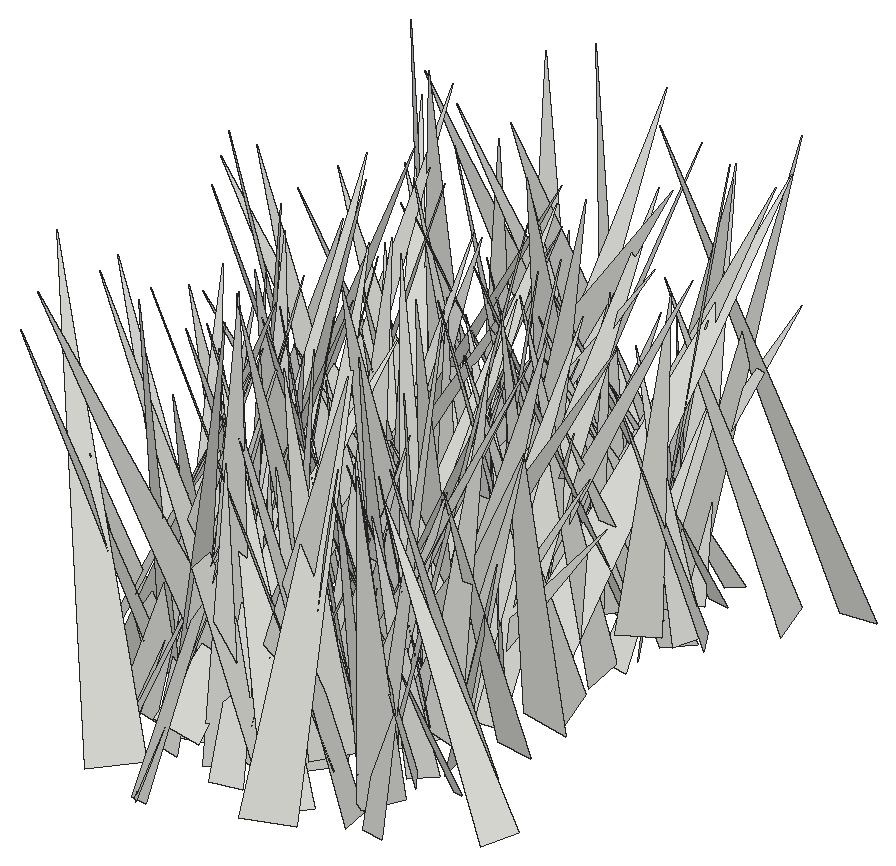
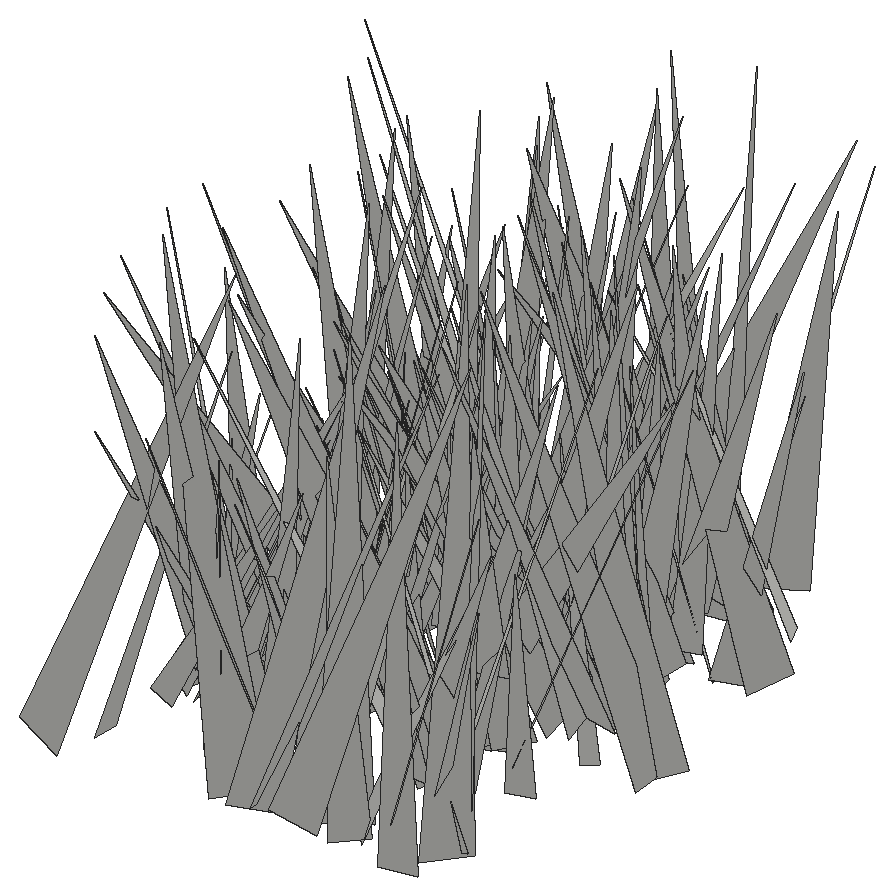
# SketchUp Ruby script. Lengths in inches.
U = 1.inch
M = Sketchup.active_model
def pt(a) = Geom::Point3d.new(a.map { |v| v * U })
def face(e, loops, mat)
  f = e.add_face(loops[0].map { |a| pt(a) })
  loops[1..].each { |l| e.add_face(l.map { |a| pt(a) }).erase! }
  f.material = f.back_material = mat if mat
  f
end
# faces: each face lists its corners as indices into pts; further lists are holes
def faces(e, pts, list, mat = nil) = list.each { |f| face(e, (f[0].is_a?(Array) ? f : [f]).map { |l| l.map { |i| pts[i] } }, mat) }
# xy, xz, yz: faces in a plane at the given z, y or x. An outline is a flat list of corners, or four numbers for a rectangle; further outlines are holes
def ring(l) = l.size == 4 ? [[l[0], l[1]], [l[2], l[1]], [l[2], l[3]], [l[0], l[3]]] : l.each_slice(2).to_a
def flat(e, list, mat, &to3) = list.each { |f| face(e, (f[0].is_a?(Array) ? f : [f]).map { |l| ring(l).map { |u, v| to3.(u, v) } }, mat) }
def xy(e, z, list, mat = nil) = flat(e, list, mat) { |x, y| [x, y, z] }
def xz(e, y, list, mat = nil) = flat(e, list, mat) { |x, z| [x, y, z] }
def yz(e, x, list, mat = nil) = flat(e, list, mat) { |y, z| [x, y, z] }
def lines(e, pts, list) = list.each { |a, b| e.add_line(pt(pts[a]), pt(pts[b])) }
# prism: a flat outline (further loops are holes) pulled along v
def prism(e, loops, v, mat = nil)
  f = face(e, loops, mat); d = Geom::Vector3d.new(v.map { |x| x * U })
  f.pushpull(f.normal.samedirection?(d) ? d.length : -d.length)
end
def box(e, o, s, mat = nil) = prism(e, [[o, [o[0] + s[0], o[1], o[2]], [o[0] + s[0], o[1] + s[1], o[2]], [o[0], o[1] + s[1], o[2]]]], [0, 0, s[2]], mat)
def at(x, y, z, deg = 0) = Geom::Transformation.translation(pt([x, y, z])) * Geom::Transformation.rotation(ORIGIN, Z_AXIS, deg.degrees)
def axes(o, x, y, z) = Geom::Transformation.new([*x, 0, *y, 0, *z, 0, *pt(o).to_a, 1])
def part(name) = M.definitions.add(name)
# library, detail: a bought-in or finely detailed component or shape, given as its bounding box
def library(name, o, s) = part(name).tap { |d| box(d.entities, o, s) }
def detail(e, o, s) = box(e.add_group.entities, o, s)
def put(e, d, t, mat = nil) = e.add_instance(d, t).tap { |i| i.material = mat if mat }
def group(e, t, mat = nil) = e.add_group.tap { |g| g.transformation = t; g.material = mat if mat }.entities
root = M.entities
c1 = part("fur_instance\#9")
p = [[0.8125,0,1.79],[0.67,-0.02,1.48],[0,-0.11,0],[0,0.11,0]]
faces(c1.entities,p,[[0,1,2,3]])
put(root,c1,axes([88.71,113.59,-28.22],[3.36953,-3.09183,0.80409],[-2.80421,-3.42236,-1.4084],[-1.53048,-0.53643,4.35081]))
put(root,c1,axes([89.1875,126.13,-28.22],[-3.67755,-0.2078,1.11626],[-0.0694,3.8179,0.48208],[1.13331,-0.4405,3.65173]))
put(root,c1,axes([89.17,122.14,-28.22],[-1.55614,3.71904,0.91385],[3.82438,1.56093,0.15988],[0.20123,-0.90564,4.0283]))
put(root,c1,axes([90.7,112.91,-27.1],[-5.38349,2.8617,0.60302],[2.91403,5.35589,0.59819],[0.24775,-0.81245,6.06741]))
put(root,c1,axes([90.85,108.57,-28.22],[-5.24663,5.623,0.95369],[5.70188,5.20042,0.70642],[0.12741,-1.17997,7.65808]))
put(root,c1,axes([88.99,124.78,-27.1],[-4.49865,-5.44108,2.87885],[-5.83326,4.90701,0.15896],[1.96626,2.10876,7.05818]))
put(root,c1,axes([90.92,124.77,-27.1],[-2.13288,4.47426,0.69403],[4.36785,1.83113,1.61826],[-1.19274,-1.2953,4.68502]))
put(root,c1,axes([86.76,118.93,-28.22],[5.41416,-4.66063,0.97473],[-4.76032,-5.26587,1.26282],[0.1044,1.59183,7.03135]))
put(root,c1,axes([89.56,112.2,-27.1],[-5.06426,-4.56399,0.84014],[-4.29824,5.08189,1.69768],[1.74956,-0.72593,6.60262]))
put(root,c1,axes([89.875,124.81,-28.22],[-5.39374,-4.42373,0.73063],[-4.15874,5.36317,1.77113],[1.67573,-0.92879,6.74722]))
put(root,c1,axes([89.88,126.89,-27.1],[-3.92886,-2.51502,0.86647],[-2.44083,4.02285,0.60923],[1.05758,-0.05874,4.62495]))
put(root,c1,axes([86.84,119.02,-28.22],[7.79072,-0.23447,0.87822],[-0.35324,-7.76347,1.06082],[-0.83754,1.09323,7.72172]))
put(root,c1,axes([92.92,120.51,-28.22],[-4.16636,5.9481,1.52453],[5.74666,3.12806,3.50054],[-2.16332,-3.14611,6.36276]))
put(root,c1,axes([91.7,117.82,-27.1],[-6.3033,-3.29184,1.05702],[-3.45211,6.11366,-1.54635],[0.19083,1.86335,6.94094]))
put(root,c1,axes([90.43,120.77,-28.22],[-5.31145,-3.30369,0.30508],[-3.10318,5.15062,1.7494],[1.17379,-1.33255,6.00546]))
put(root,c1,axes([88.53,117.63,-28.22],[6.37942,2.61315,2.43113],[3.05762,-6.56979,-0.96169],[-1.84118,-1.85616,6.82648]))
put(root,c1,axes([91.35,126.52,-28.22],[-3.75562,-3.58045,0.3486],[-3.58145,3.67402,-0.84892],[-0.33818,0.85312,5.11895]))
put(root,c1,axes([88.83,119.2,-27.1],[1.55056,7.17303,0.47228],[7.18686,-1.53634,-0.26142],[0.15632,-0.51668,7.33405]))
put(root,c1,axes([89.91,115.51,-28.22],[2.88835,4.68484,1.93004],[4.79823,-3.24275,0.69058],[-1.62782,-1.24585,5.46016]))
put(root,c1,axes([88.52,126.21,-28.22],[7.55718,-3.05255,1.8054],[-2.7949,-7.74218,-1.39129],[-2.18313,-0.65505,8.03077]))
put(root,c1,axes([90.47,115.76,-28.22],[3.4747,-4.84053,2.29693],[-4.84614,-4.00697,-1.11322],[-2.28507,1.13736,5.85363]))
put(root,c1,axes([88.5,125.73,-28.22],[-0.2038,-3.57727,1.86557],[-3.68837,0.92217,1.36537],[1.63497,1.63446,3.31273]))
put(root,c1,axes([91.42,120.62,-28.22],[-3.35316,6.39569,0.22234],[6.39729,3.34326,0.30873],[-0.17041,-0.34016,7.2148]))
put(root,c1,axes([90.11,116.29,-28.22],[-2.28357,5.70644,2.33564],[6.0895,2.47813,-0.10083],[0.96778,-2.12809,6.14557]))
put(root,c1,axes([89.13,127.62,-28.22],[0.11264,-6.37998,1.60761],[-6.5012,0.13924,1.0081],[1.01142,1.60553,6.30084]))
put(root,c1,axes([91.64,122.14,-27.1],[-5.50696,2.25656,1.40845],[2.52369,5.45565,1.12666],[0.84072,-1.59571,5.84374]))
put(root,c1,axes([87.69,111.89,-27.1],[5.0651,3.0377,0.15182],[3.00547,-4.95362,-1.15532],[0.46672,-1.0677,5.79207]))
put(root,c1,axes([90.78,122.63,-28.22],[-1.67954,-4.60165,1.09216],[-4.72861,1.65608,-0.29411],[0.09072,1.12742,4.88974]))
put(root,c1,axes([92.49,117.92,-27.1],[0.18988,-6.4583,3.19895],[-6.79344,-1.22898,-2.07794],[-2.40669,2.95955,6.11783]))
put(root,c1,axes([89.45,114.52,-27.1],[-0.0268,-5.65268,0.22398],[-5.53849,0.07185,1.15049],[1.15241,0.21383,5.53443]))
put(root,c1,axes([87.68,112.9375,-28.22],[7.43524,-1.67911,0.29476],[-1.69435,-7.42416,0.44731],[-0.18841,0.50147,7.60934]))
put(root,c1,axes([91.88,128.85,-27.1],[0.79588,-7.21699,0.96951],[-7.03929,-1.01213,-1.75565],[-1.86367,0.74092,7.04528]))
put(root,c1,axes([89.52,113.33,-28.22],[4.5925,4.65986,1.11021],[4.70947,-4.6734,0.13435],[-0.87619,-0.69491,6.5412]))
put(root,c1,axes([88.76,119.6,-28.22],[4.69242,0.16576,0.10905],[0.19618,-4.2622,-1.96297],[-0.02968,-1.96577,4.26532]))
put(root,c1,axes([92.05,112.9,-27.1],[1.02305,5.31057,1.33507],[5.15193,-1.39366,1.59576],[-1.8553,-0.94167,5.16743]))
put(root,c1,axes([89.0625,119.71,-27.1],[6.34041,1.92452,0.88463],[1.94009,-6.39712,0.01179],[-0.84995,-0.24555,6.62604]))
put(root,c1,axes([91.54,110.98,-28.22],[-1.61925,6.67608,1.38838],[6.8184,1.60284,0.24489],[0.08425,-1.4073,6.86528]))
put(root,c1,axes([91.35,110.12,-28.22],[2.76869,6.15296,0.77217],[6.00563,-2.8712,1.34513],[-1.54517,-0.13446,6.61174]))
put(root,c1,axes([93.52,111.33,-27.1],[0.24896,-7.3468,1.55373],[-6.97419,-0.80255,-2.67734],[-2.78393,1.35351,6.84612]))
put(root,c1,axes([90.86,113.59,-28.22],[-1.14842,8.02715,0.79991],[8.02073,1.22255,-0.75306],[0.86188,-0.68125,8.07384]))
put(root,c1,axes([89.41,111.35,-28.22],[1.22983,-5.08709,1.30795],[-5.046,-0.77126,1.74491],[1.45845,1.62123,4.93419]))
put(root,c1,axes([90.24,111.79,-27.1],[-3.33298,-6.74445,1.96036],[-6.484,3.7887,2.01069],[2.69971,0.77298,7.24938]))
put(root,c1,axes([89,115.69,-27.1],[6.32916,0.13104,0.27334],[0.13733,-6.3333,-0.14369],[-0.27023,-0.14945,6.32889]))
put(root,c1,axes([89.87,115.43,-28.22],[7.83085,1.1219,1.78667],[1.00117,-8.02181,0.64907],[-1.85702,0.40616,7.88414]))
put(root,c1,axes([89.28,111.27,-28.22],[5.01329,4.55618,1.17415],[4.70331,-4.80639,-1.43108],[0.12753,-1.84671,6.62147]))
put(root,c1,axes([89.94,116.67,-28.22],[6.05752,-0.57817,0.88939],[-0.39,-6.0087,-1.2499],[-0.9865,-1.17476,5.9553]))
put(root,c1,axes([90.48,117.5,-27.1],[4.1786,-6.03386,0.40804],[-6.0035,-4.19846,-0.60465],[-0.72937,-0.01047,7.31455]))
put(root,c1,axes([91.7,114.43,-28.22],[-3.27969,0.65416,1.38528],[0.68941,3.5533,-0.04576],[1.36808,-0.22237,3.34398]))
put(root,c1,axes([90.06,109.9,-28.22],[3.49532,2.40186,0.16337],[2.40303,-3.46356,-0.49202],[0.14512,-0.49771,4.21237]))
put(root,c1,axes([89.8,121.63,-27.1],[3.48254,-4.50934,1.30252],[-4.66936,-3.1635,1.53235],[0.47726,1.95368,5.48763]))
put(root,c1,axes([92.99,120.28,-27.1],[-4.59731,-1.23154,0.33008],[-1.08177,4.4213,1.42926],[0.67485,-1.30242,4.53973]))
put(root,c1,axes([89.44,117.55,-28.22],[2.82226,4.09729,0.68802],[3.94816,-2.38599,-1.98631],[1.29353,-1.65697,4.56152]))
put(root,c1,axes([93.32,128.47,-27.1],[-6.61379,-2.13915,0.88077],[-1.88588,6.53057,1.69974],[1.33985,-1.36736,6.74011]))
put(root,c1,axes([92,126.45,-28.22],[4.03772,-5.94106,3.0996],[-6.44975,-4.42725,-0.08397],[-1.8178,2.512,7.18278]))
put(root,c1,axes([95.09,110.51,-28.22],[-7.85705,-0.88135,0.16267],[-0.88597,7.85465,-0.23661],[0.1352,0.25331,7.90278]))
put(root,c1,axes([93.91,113.9,-28.22],[-2.37076,-5.83706,1.32394],[-5.9146,2.06646,-1.48049],[-0.91737,1.76156,6.12372]))
put(root,c1,axes([91.4,117.29,-27.1],[-2.96228,-3.48582,0.87467],[-2.85625,2.97145,2.16874],[2.18125,-0.843,4.02773]))
put(root,c1,axes([91.25,126.54,-28.22],[3.73813,0.01426,0.67221],[0.17612,-3.68545,-0.90117],[-0.64889,-0.91811,3.62791]))
put(root,c1,axes([89.66,119.66,-27.1],[7.04502,0.38941,0.11832],[0.34745,-6.82295,1.76766],[-0.21195,1.75889,6.83077]))
put(root,c1,axes([92.1,114.49,-28.22],[-0.97227,-5.54065,0.71566],[-5.53732,1.05209,0.62249],[0.741,0.5921,5.59077]))
put(root,c1,axes([91.26,127.08,-28.22],[3.84963,-3.94903,0.87916],[-4.01863,-3.87266,0.20133],[-0.4673,0.77142,5.51126]))
put(root,c1,axes([92.59,107.42,-28.22],[4.07419,5.57288,0.07978],[5.18286,-3.82462,2.48447],[-2.04971,1.40628,6.44076]))
put(root,c1,axes([92.25,121.4,-28.22],[4.66089,-0.94094,1.87831],[-0.93791,-5.02216,-0.1885],[-1.87983,0.17273,4.75118]))
put(root,c1,axes([92.02,116.3125,-28.22],[2.22729,6.28936,0.04999],[6.2767,-2.22605,0.40869],[-0.40191,0.08939,6.65956]))
put(root,c1,axes([90.33,117.78,-27.1],[6.45135,0.1489,0.38361],[-0.04006,-5.77049,2.9136],[-0.40954,2.91007,5.75787]))
put(root,c1,axes([90.03,123.73,-27.1],[5.30447,3.34271,0.68413],[3.37643,-4.96043,-1.94241],[0.49141,-1.99988,5.96139]))
put(root,c1,axes([92.61,126.5,-28.22],[-3.5223,-6.70382,0.02091],[-6.50166,3.42181,1.83516],[1.63401,-0.83562,7.34711]))
put(root,c1,axes([92.48,107.4,-28.22],[3.00596,2.69315,0.13963],[2.45938,-2.82346,1.51258],[-1.10635,1.04086,3.74179]))
put(root,c1,axes([93.52,117.36,-28.22],[-3.36286,5.21282,1.50099],[5.38655,3.41774,0.19865],[0.64152,-1.37145,6.20023]))
put(root,c1,axes([94.96,120.65,-27.1],[-6.17227,-0.98801,0.5453],[-1.07692,6.06305,-1.2042],[0.3373,1.27815,6.13375]))
put(root,c1,axes([91.98,120.85,-28.22],[0.60186,-6.09784,0.10298],[-6.0697,-0.58883,0.60707],[0.59415,0.16161,6.09732]))
put(root,c1,axes([94.66,115.76,-27.1],[-4.58981,-6.81856,1.14154],[-6.9132,4.53833,-0.68805],[0.05895,1.33156,8.19058]))
put(root,c1,axes([90.97,111.66,-27.1],[7.66875,0.29762,1.40281],[0.64374,-7.5341,-1.92071],[-1.28143,-2.00373,7.43029]))
put(root,c1,axes([92.23,111.7,-28.22],[1.05516,-7.50337,2.43147],[-7.87164,-0.84629,0.8044],[0.49989,2.51181,7.53438]))
put(root,c1,axes([93.2,128.94,-27.1],[6.13444,-4.45258,1.42838],[-3.84619,-6.14459,-2.6359],[-2.65943,-1.38408,7.10696]))
put(root,c1,axes([92.78,116.5,-28.22],[4.75602,-4.66812,2.75377],[-5.20371,-4.95731,0.58378],[-1.51526,2.37234,6.63855]))
put(root,c1,axes([93.22,110.32,-28.22],[2.46407,-3.91283,1.91735],[-4.25122,-2.64198,0.07181],[-0.95581,1.66367,4.6235]))
put(root,c1,axes([92.98,112.73,-27.1],[4.79862,3.05458,1.6678],[3.017,-5.06719,0.60002],[-1.73486,-0.36311,5.65661]))
put(root,c1,axes([93.94,109.59,-28.22],[-0.89857,4.82904,0.37817],[4.8418,0.88433,0.21213],[-0.14006,-0.41036,4.90735]))
put(root,c1,axes([96.81,110.76,-27.1],[-5.69424,-4.56861,0.52497],[-4.47673,5.31586,-2.29625],[-1.05201,2.10752,6.92992]))
put(root,c1,axes([92.21,109.55,-27.1],[-1.93127,6.17376,0.09606],[5.65668,1.80943,-2.5656],[2.47519,0.68189,5.93825]))
put(root,c1,axes([93.39,117.71,-28.22],[4.88269,3.53574,0.69101],[3.04894,-4.67553,2.3797],[-1.91908,1.56767,5.53887]))
put(root,c1,axes([93.85,116.83,-28.22],[3.06348,4.37723,2.06786],[4.6001,-3.39453,0.37061],[-1.50841,-1.46222,5.32989]))
put(root,c1,axes([93.46,111.42,-27.1],[5.52585,4.05046,1.31825],[3.69086,-5.63091,1.83015],[-2.12639,0.75214,6.60241]))
put(root,c1,axes([96.24,109.55,-28.22],[-3.04335,5.85133,0.32291],[5.70958,2.87864,1.64877],[-1.32023,-1.03909,6.38604]))
put(root,c1,axes([94.43,123.98,-28.22],[-4.52954,-3.25843,1.35312],[-3.24257,4.71245,0.49358],[1.39071,0.3748,5.55792]))
put(root,c1,axes([94.77,114.29,-28.22],[-4.49464,-4.79472,1.8462],[-5.03521,4.59856,-0.3156],[1.02201,1.56958,6.56442]))
put(root,c1,axes([92.94,122,-27.1],[3.65052,-1.24636,0.3015],[-1.17659,-3.61738,-0.70767],[-0.50984,-0.576,3.79195]))
put(root,c1,axes([94.66,118.05,-27.1],[0.91416,-4.94391,1.27953],[-4.9749,-1.15567,-0.91103],[-1.1532,1.06645,4.94449]))
put(root,c1,axes([96.16,121.2,-27.1],[-6.23091,-2.8217,1.23434],[-3.03851,6.08694,-1.42355],[0.50305,1.81577,6.69027]))
put(root,c1,axes([95.5,121.05,-28.22],[-4.37438,2.14658,0.79892],[2.22863,4.38643,0.41683],[0.52851,-0.72986,4.85482]))
put(root,c1,axes([94.77,113.72,-28.22],[-0.40917,-7.70862,1.45343],[-7.84037,0.35495,-0.32469],[-0.25296,1.46762,7.71264]))
put(root,c1,axes([93.57,117.34,-27.1],[-1.05391,6.67902,0.37292],[6.52998,1.10912,-1.41007],[1.4518,-0.14015,6.613]))
put(root,c1,axes([90.14,124.27,-27.1],[3.5795,-7.50714,1.0436],[-6.77337,-2.6505,4.166],[3.40115,2.62237,7.19823]))
put(root,c1,axes([95.68,122.73,-28.22],[-1.02707,-3.52995,0.46815],[-3.49734,0.90838,-0.82343],[-0.66956,0.66999,3.58293]))
put(root,c1,axes([95.625,120.07,-28.22],[-4.12735,0.23871,1.0618],[0.66209,3.85593,1.70672],[0.86374,-1.81501,3.76552]))
put(root,c1,axes([94.02,111.16,-28.22],[3.84867,2.11329,0.22175],[1.92609,-3.66331,1.48248],[-0.8974,1.20066,4.13285]))
put(root,c1,axes([93.49,125.47,-27.1],[6.57894,-4.30915,0.69378],[-4.10201,-6.53322,-1.6802],[-1.49116,-1.03963,7.68298]))
put(root,c1,axes([95.58,110.25,-27.1],[-5.55203,-0.57439,2.02149],[-1.15794,5.60149,-1.58866],[1.75372,1.88009,5.3508]))
put(root,c1,axes([96.48,119.68,-27.1],[-4.58917,0.765,0.19448],[0.68534,4.43094,-1.25723],[0.3916,1.21042,4.47941]))
put(root,c1,axes([95.26,111.75,-28.22],[3.00214,-3.52749,1.91618],[-3.65397,-3.39209,-0.51969],[-1.66236,1.08552,4.60282]))
put(root,c1,axes([97.95,110.26,-28.22],[-6.99068,-2.50094,0.47101],[-2.54423,6.83653,-1.46112],[-0.05835,1.53405,7.27938]))
put(root,c1,axes([93.89,113.8,-28.22],[2.56604,4.25646,1.10853],[4.39439,-2.42581,-0.85772],[0.18887,-1.38883,4.89555]))
put(root,c1,axes([93.77,120.16,-27.1],[2.51167,3.62255,0.80621],[3.69421,-2.34748,-0.96099],[0.35452,-1.20325,4.30208]))
put(root,c1,axes([91.45,121.78,-27.1],[4.41498,5.25807,0.18984],[4.81628,-3.93899,-2.90917],[2.11822,-2.00311,6.21901]))
put(root,c1,axes([94.46,120.72,-27.1],[-4.73234,6.09922,1.47861],[5.53404,4.92888,-2.61961],[2.95993,0.53615,7.26177]))
put(root,c1,axes([94.48,117.12,-27.1],[5.05065,-5.78899,0.88016],[-5.66798,-5.12516,-1.18448],[-1.47008,-0.1285,7.59069]))
put(root,c1,axes([93.85,125.09,-27.1],[3.11489,-2.67244,0.85057],[-2.80172,-2.90834,1.1224],[0.12545,1.40269,3.94774]))
put(root,c1,axes([97.53,122.43,-27.1],[-7.91635,-0.39433,1.24518],[-0.80795,7.48837,-2.76517],[1.02625,2.85367,7.42819]))
put(root,c1,axes([94.41,124.13,-27.1],[3.13129,2.44329,0.37399],[2.42945,-3.15346,0.26073],[-0.45532,-0.0231,3.96316]))
put(root,c1,axes([94.34,116.88,-28.22],[3.7464,3.46532,0.67043],[3.46985,-3.79505,0.22613],[-0.64655,-0.28736,5.09832]))
put(root,c1,axes([93.67,121.89,-28.22],[5.80303,5.01805,0.27093],[4.96083,-5.78629,0.91567],[-0.80277,0.51711,7.61693]))
put(root,c1,axes([96.18,112.01,-28.22],[2.91558,3.30379,0.88214],[2.68077,-2.92801,2.10571],[-2.12289,0.83996,3.8706]))
put(root,c1,axes([96.7,114.85,-28.22],[-6.58758,2.43197,1.48528],[2.355,6.75255,-0.6115],[1.60454,0.07391,6.99549]))
put(root,c1,axes([94.44,119.86,-27.1],[3.52648,2.43175,0.31475],[2.41999,-3.54045,0.23962],[-0.3951,0.0194,4.27692]))
put(root,c1,axes([95.7,125.25,-27.1],[-1.12897,-3.54048,0.33773],[-3.515,1.16474,0.46018],[0.54205,0.17891,3.68752]))
put(root,c1,axes([95.87,114.5,-27.1],[-4.47907,3.89554,0.463],[3.44419,4.24137,-2.36643],[1.87807,1.51235,5.44401]))
put(root,c1,axes([96.28,113.34,-27.1],[1.74245,-3.02379,2.07472],[-3.3962,-2.19711,-0.34987],[-1.38332,1.58534,3.47232]))
put(root,c1,axes([94.8,115.85,-28.22],[-1.97553,-6.78705,1.45707],[-6.65434,2.28292,1.61176],[1.97656,0.90224,6.88251]))
put(root,c1,axes([97.3,125.2,-27.1],[-3.1283,2.85302,0.75954],[2.94685,2.94951,1.058],[-0.18092,-1.28978,4.09959]))
put(root,c1,axes([93.88,110.88,-28.22],[1.0853,-7.02468,2.48253],[-7.23303,-0.3918,2.05344],[1.78669,2.68091,6.80495]))
put(root,c1,axes([96.5,111.15,-27.1],[-4.53938,3.59005,2.40826],[4.08452,4.7056,0.68422],[1.41595,-2.06469,5.74685]))
put(root,c1,axes([96.88,119.66,-27.1],[-4.48858,-3.56813,1.07524],[-3.58767,4.5928,0.2643],[1.00813,0.45789,5.72792]))
put(root,c1,axes([96.57,115.45,-27.1],[-2.51428,-3.3921,0.48717],[-3.39486,2.54791,0.21985],[0.4675,0.25907,4.21659]))
put(root,c1,axes([97.39,107.13,-27.1],[-7.03666,4.34174,0.35439],[3.96979,6.66848,-2.87454],[1.79361,2.2741,7.75256]))
put(root,c1,axes([96,115.6,-27.1],[-2.86919,-3.90872,1.79506],[-4.01549,3.2075,0.56601],[1.54149,1.08002,4.8156]))
put(root,c1,axes([93.5625,115.74,-28.22],[7.09843,0.26187,0.16049],[0.26265,-7.10014,-0.03187],[-0.15921,-0.03777,7.10319]))
put(root,c1,axes([95.84,121.8,-28.22],[2.50338,-2.82714,1.30611],[-3.05988,-2.54469,0.35667],[-0.57944,1.22368,3.75931]))
put(root,c1,axes([97.56,111.18,-27.1],[-5.21816,-1.76906,1.50642],[-2.07355,5.2165,-1.05669],[1.04846,1.51216,5.4076]))
put(root,c1,axes([96,117.41,-28.22],[4.06792,5.19434,1.22411],[5.14399,-4.22635,0.83955],[-1.42088,-0.42943,6.54403]))
put(root,c1,axes([95.24,117.55,-27.1],[-0.53699,-7.34105,1.16615],[-7.27133,0.76139,1.44476],[1.5423,1.0337,7.21748]))
put(root,c1,axes([94.66,125.84,-28.22],[3.70587,4.25797,0.60198],[4.28884,-3.60158,-0.92773],[0.31394,-1.06043,5.56805]))
put(root,c1,axes([95.83,110.22,-27.1],[3.79573,2.84609,1.46317],[3.05532,-3.89817,-0.34352],[-0.95191,-1.16307,4.73179]))
put(root,c1,axes([95.26,120.61,-28.22],[4.21997,-0.6182,0.41958],[-0.60999,-4.24047,-0.11271],[-0.43142,-0.05127,4.26352]))
put(root,c1,axes([96.29,126.54,-28.22],[3.50873,2.55931,1.93983],[3.03472,-3.58228,-0.76287],[-1.05048,-1.80039,4.27543]))
put(root,c1,axes([97.21,114.46,-27.1],[2.58883,2.26123,2.35644],[2.87323,-3.00647,-0.27159],[-1.55259,-1.79333,3.42658]))
put(root,c1,axes([95.36,120.72,-27.1],[6.75458,-3.1446,1.55563],[-3.25939,-6.87331,0.25842],[-1.29802,0.89549,7.44621]))
put(root,c1,axes([99.4,124.56,-27.1],[-2.79932,-5.24784,0.26282],[-5.09915,2.64134,-1.57068],[-1.26789,0.96362,5.73663]))
put(root,c1,axes([97.33,125.81,-28.22],[-2.49049,-3.07283,1.62396],[-3.33154,2.67981,-0.03854],[0.99012,1.28779,3.95516]))
put(root,c1,axes([97.47,121.35,-27.1],[1.36793,4.62634,1.5435],[4.80198,-1.5578,0.41343],[-0.85231,-1.35162,4.8066]))
put(root,c1,axes([99.24,113.23,-28.22],[-2.45268,-3.25533,0.28731],[-3.08329,2.18606,-1.55237],[-1.08306,1.14864,3.76868]))
put(root,c1,axes([97.01,116.69,-28.22],[-5.76444,5.45156,1.05869],[4.71185,5.60881,-3.22628],[2.93919,1.70025,7.24841]))
put(root,c1,axes([98.35,125,-27.1],[-4.30266,-2.43803,0.04686],[-2.30354,4.09498,1.544],[0.79994,-1.32144,4.69819]))
put(root,c1,axes([98.8,123.53,-28.22],[0.61294,-5.47928,1.38132],[-5.30961,-1.0339,-1.7451],[-1.93355,1.10218,5.22999]))
put(root,c1,axes([97.9375,122.34,-27.1],[-3.38776,-6.42257,0.32475],[-6.36234,3.40084,0.88702],[0.93573,-0.12917,7.20691]))
put(root,c1,axes([98.23,120.91,-28.22],[-6.02473,-0.71032,1.74625],[-0.51818,6.24626,0.75302],[1.81257,-0.57532,6.01954]))
put(root,c1,axes([97.92,113.35,-28.22],[1.60844,-3.68609,1.55705],[-3.78668,-1.94455,-0.69177],[-1.29334,1.10916,3.96179]))
put(root,c1,axes([97.56,117.29,-27.1],[2.96101,1.91002,1.7712],[2.18546,-3.28075,-0.11568],[-1.41742,-1.06838,3.5217]))
put(root,c1,axes([95.72,125.45,-27.1],[2.4486,-4.30122,0.69777],[-4.269,-2.2075,1.37318],[0.8735,1.26866,4.75506]))
put(root,c1,axes([95.25,126.93,-28.22],[5.39011,-5.98506,0.75501],[-6.02641,-5.29691,1.03406],[0.27067,1.25142,7.9878]))
put(root,c1,axes([94.82,114.72,-27.1],[6.0574,2.72005,0.2303],[2.69232,-5.86042,-1.5971],[0.45071,-1.54939,6.44516]))
put(root,c1,axes([96.69,116.01,-28.22],[0.10942,6.44965,1.02032],[6.44115,0.06102,-1.07648],[1.07264,-1.02435,6.36012]))
put(root,c1,axes([95.84,118.36,-27.1],[2.51119,2.94201,0.30611],[2.79372,-2.22715,-1.51331],[0.97173,-1.19981,3.55969]))
put(root,c1,axes([99.17,125.57,-27.1],[-0.33006,-3.76044,0.39687],[-3.50265,0.15395,-1.45434],[-1.42474,0.49269,3.4835]))
put(root,c1,axes([96.31,112.94,-27.1],[3.07396,-3.53335,0.83024],[-3.61315,-2.87553,1.13994],[0.34489,1.36741,4.5425]))
put(root,c1,axes([98.84,109.9375,-28.22],[3.53249,6.50702,1.2231],[6.07163,-3.73652,2.34297],[-2.64057,0.11331,7.02355]))
put(root,c1,axes([95.13,122.7,-28.22],[2.59444,7.48207,1.23534],[7.31718,-2.12705,-2.48457],[1.99156,-1.93206,7.51927]))
put(root,c1,axes([98.56,122.62,-27.1],[0.67909,-3.62862,0.46379],[-3.53581,-0.77205,-0.86319],[-0.93808,0.2832,3.58928]))
put(root,c1,axes([98.83,118.92,-28.22],[-5.96376,-1.66281,1.60864],[-1.32131,6.09893,1.40577],[1.89916,-0.97833,6.02952]))
put(root,c1,axes([95.04,115.85,-27.1],[6.3813,-2.25892,0.20905],[-2.20352,-6.02357,2.17449],[0.53935,2.11689,6.41056]))
put(root,c1,axes([99.08,111.58,-27.1],[-3.66395,-2.75565,0.79106],[-2.79858,3.7164,-0.01609],[0.62239,0.48852,4.58453]))
put(root,c1,axes([96.05,124.03,-28.22],[1.81357,5.35205,0.20733],[5.12174,-1.66889,-1.72019],[1.56691,-0.73948,5.38279]))
put(root,c1,axes([97.84,115.16,-27.1],[-4.49953,-3.59508,3.80394],[-4.60675,5.10137,-0.62788],[2.48443,2.94818,5.72505]))
put(root,c1,axes([98.67,123.78,-27.1],[-5.11212,3.73872,1.49873],[3.53116,5.32488,-1.23875],[1.93782,0.15985,6.21106]))
put(root,c1,axes([98,124.37,-27.1],[3.54062,0.10617,1.20258],[0.38468,-3.63127,-0.812],[-1.14433,-0.89222,3.44788]))
put(root,c1,axes([95.1,120.63,-27.1],[5.1253,5.35023,0.94765],[5.22805,-4.50107,-2.86349],[1.48003,-2.62814,6.83331]))
put(root,c1,axes([98.1,121.5,-28.22],[-0.08905,4.06249,0.07241],[4.03019,0.09752,-0.5148],[0.51634,-0.06053,4.03072]))
put(root,c1,axes([96.73,114.79,-27.1],[4.08139,-3.20586,0.61223],[-3.2526,-3.91407,1.18774],[0.27008,1.30866,5.05219]))
put(root,c1,axes([98,111.38,-28.22],[4.8862,-3.80667,1.31151],[-3.74132,-5.05482,-0.73291],[-1.48774,0.20937,6.1505]))
put(root,c1,axes([97.79,111.97,-27.1],[6.38887,5.18246,1.59043],[5.07791,-6.58181,1.04866],[-1.89794,-0.16426,8.1594]))
put(root,c1,axes([96.32,118.09,-27.1],[2.45066,3.05169,0.44917],[2.65928,-1.79957,-2.28257],[1.56295,-1.7231,3.17938]))
put(root,c1,axes([97.22,119.48,-27.1],[-2.37553,7.32496,0.20013],[6.77476,2.27563,-2.87444],[2.79244,0.71043,7.14393]))
put(root,c1,axes([94.87,113.52,-27.1],[7.11507,4.33314,0.48127],[4.20256,-6.57141,-2.9643],[1.16029,-2.76992,7.78545]))
put(root,c1,axes([98.68,123.56,-27.1],[6.48387,0.57283,2.72889],[-0.5216,-6.53637,2.61139],[-2.73914,2.60063,5.96233]))
put(root,c1,axes([98.68,117.78,-28.22],[-0.69172,-7.26259,1.83893],[-7.46362,0.82804,0.46276],[0.64909,1.78171,7.28077]))
put(root,c1,axes([98.21,114.24,-28.22],[3.55375,0.65284,0.74182],[0.70307,-3.6162,-0.18565],[-0.69441,-0.32026,3.60844]))
put(root,c1,axes([97.93,122.89,-28.22],[6.38411,4.40631,2.11358],[4.61615,-6.57865,-0.22824],[-1.60436,-1.39477,7.75373]))
put(root,c1,axes([100.11,122.34,-27.1],[-4.10178,1.61092,0.95507],[1.70987,4.15942,0.32775],[0.76391,-0.66031,4.39457]))
put(root,c1,axes([98.14,113.82,-27.1],[-0.07815,-6.05054,2.52953],[-6.4447,0.53908,1.09033],[1.2138,2.47266,5.952]))
put(root,c1,axes([100.43,113.03,-27.1],[-1.57238,-4.56901,1.11948],[-4.65933,1.35009,-1.0341],[-0.64787,1.37945,4.72005]))
put(root,c1,axes([98.91,116.13,-28.22],[-0.08674,-5.50292,0.32115],[-5.49794,0.10952,0.39174],[0.3974,0.31411,5.48965]))
put(root,c1,axes([101.68,127.87,-28.22],[-2.55131,-7.67351,1.38924],[-7.65133,2.18082,-2.00574],[-1.50657,1.91917,7.83383]))
put(root,c1,axes([96.99,115.6,-27.1],[1.53835,-7.01276,2.03333],[-7.04829,-0.88366,2.28484],[1.90652,2.39168,6.80623]))
put(root,c1,axes([100.4,126.52,-28.22],[-5.81258,-1.56867,1.18702],[-1.32265,5.85738,1.26392],[1.45614,-0.94136,5.88637]))
put(root,c1,axes([101.75,111.94,-28.22],[-3.98181,3.20015,0.16473],[3.12043,3.81261,1.36007],[-0.7287,-1.16015,4.92402]))
put(root,c1,axes([98.82,121.72,-27.1],[3.55242,-4.27149,1.91187],[-4.60398,-3.6203,0.46613],[-0.83917,1.77997,5.53606]))
put(root,c1,axes([100.48,122.64,-27.1],[-3.61255,-2.36918,0.54232],[-2.35627,3.65218,0.25916],[0.59592,0.07847,4.31235]))
